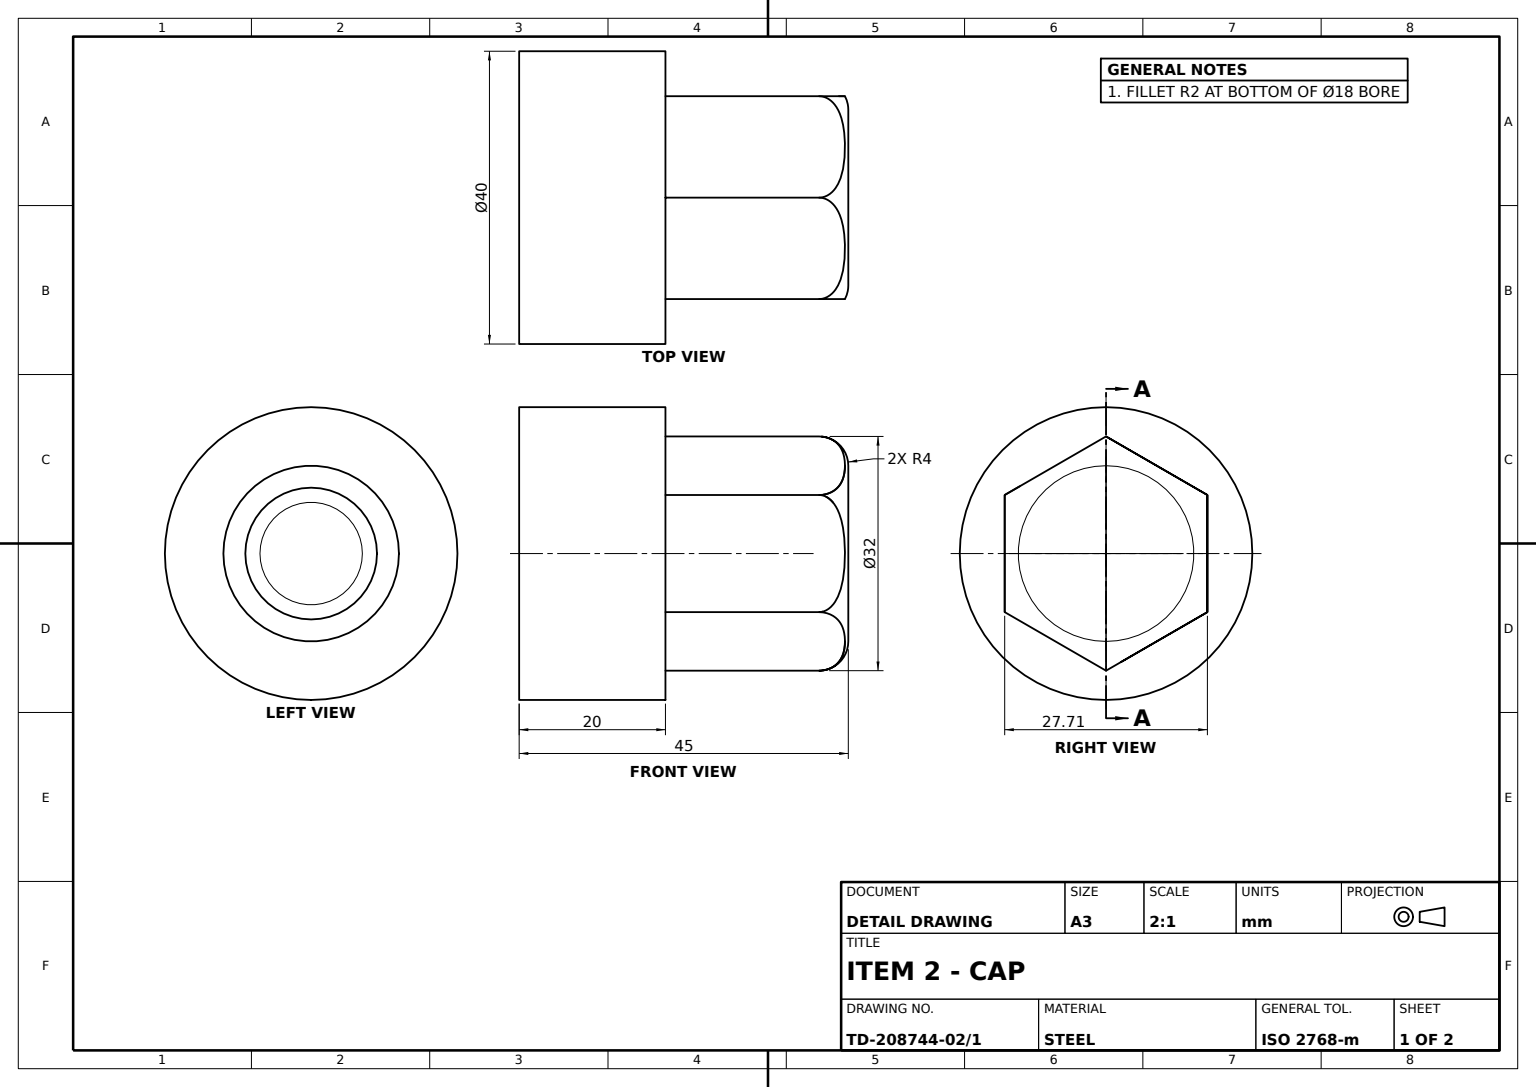
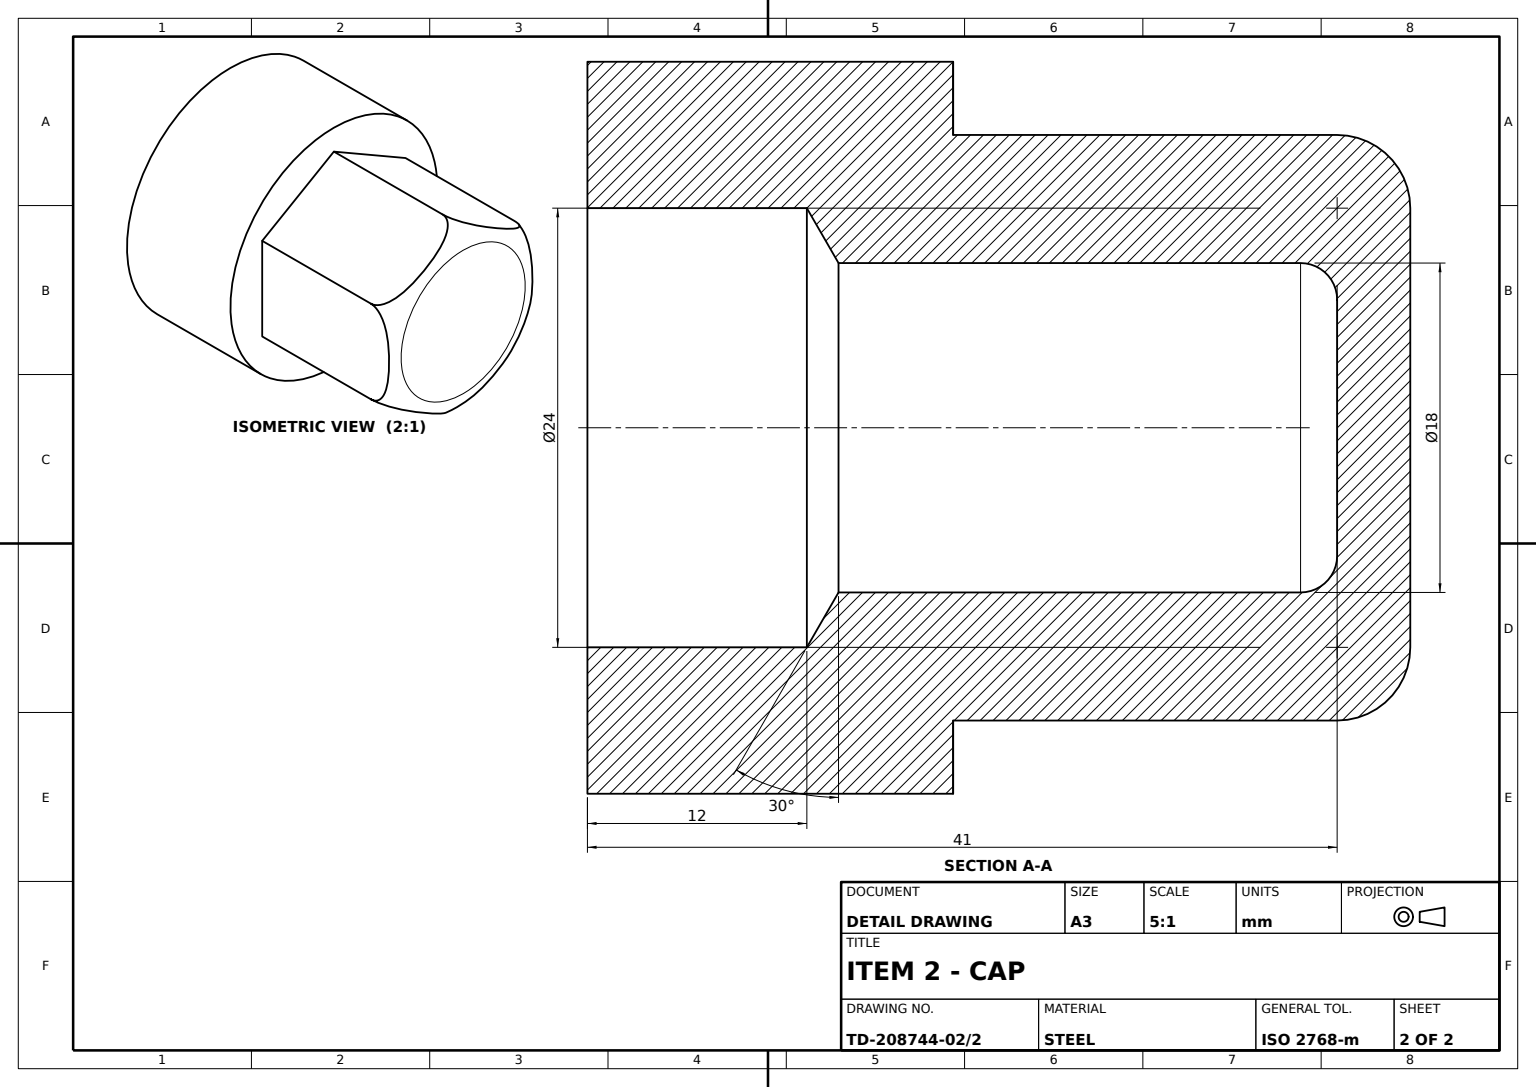
ISO-10303-21;
HEADER;
FILE_DESCRIPTION((''),'2;1');
FILE_NAME('','',(''),(''),'','','');
FILE_SCHEMA(('AUTOMOTIVE_DESIGN'));
ENDSEC;
DATA;
#1=APPLICATION_CONTEXT('');
#2=PRODUCT_CONTEXT('',#1,'mechanical');
#3=PRODUCT('','','',(#2));
#4=PRODUCT_DEFINITION_FORMATION('','',#3);
#5=PRODUCT_DEFINITION_CONTEXT('',#1,'design');
#6=PRODUCT_DEFINITION('','',#4,#5);
#7=PRODUCT_DEFINITION_SHAPE('','',#6);
#8=(LENGTH_UNIT()NAMED_UNIT(*)SI_UNIT(.MILLI.,.METRE.));
#9=(NAMED_UNIT(*)PLANE_ANGLE_UNIT()SI_UNIT($,.RADIAN.));
#10=(NAMED_UNIT(*)SI_UNIT($,.STERADIAN.)SOLID_ANGLE_UNIT());
#11=UNCERTAINTY_MEASURE_WITH_UNIT(LENGTH_MEASURE(1.E-05),#8,'distance_accuracy_value','');
#12=(GEOMETRIC_REPRESENTATION_CONTEXT(3)GLOBAL_UNCERTAINTY_ASSIGNED_CONTEXT((#11))GLOBAL_UNIT_ASSIGNED_CONTEXT((#8,#9,#10))REPRESENTATION_CONTEXT('',''));
#13=CARTESIAN_POINT('',(0.,0.,12.));
#14=VERTEX_POINT('',#13);
#15=CARTESIAN_POINT('',(0.,0.,-12.));
#16=VERTEX_POINT('',#15);
#17=CARTESIAN_POINT('',(0.,0.,0.));
#18=DIRECTION('',(0.,-1.,0.));
#19=DIRECTION('',(0.,0.,-1.));
#20=AXIS2_PLACEMENT_3D('',#17,#18,#19);
#21=CIRCLE('',#20,12.);
#22=EDGE_CURVE('',#14,#16,#21,.T.);
#23=ORIENTED_EDGE('',*,*,#22,.F.);
#24=EDGE_CURVE('',#16,#14,#21,.T.);
#25=ORIENTED_EDGE('',*,*,#24,.F.);
#26=EDGE_LOOP('',(#23,#25));
#27=FACE_BOUND('',#26,.T.);
#28=CARTESIAN_POINT('',(-20.,0.,0.));
#29=VERTEX_POINT('',#28);
#30=CARTESIAN_POINT('',(20.,0.,0.));
#31=VERTEX_POINT('',#30);
#32=DIRECTION('',(1.,0.,0.));
#33=AXIS2_PLACEMENT_3D('',#17,#18,#32);
#34=CIRCLE('',#33,20.);
#35=EDGE_CURVE('',#29,#31,#34,.T.);
#36=ORIENTED_EDGE('',*,*,#35,.T.);
#37=EDGE_CURVE('',#31,#29,#34,.T.);
#38=ORIENTED_EDGE('',*,*,#37,.T.);
#39=EDGE_LOOP('',(#36,#38));
#40=FACE_OUTER_BOUND('',#39,.T.);
#41=PLANE('',#33);
#42=ADVANCED_FACE('',(#27,#40),#41,.T.);
#43=CARTESIAN_POINT('',(0.,39.,-9.));
#44=VERTEX_POINT('',#43);
#45=CARTESIAN_POINT('',(0.,13.732051,-9.));
#46=VERTEX_POINT('',#45);
#47=CARTESIAN_POINT('',(0.,0.,-9.));
#48=VECTOR('',#18,1000.);
#49=LINE('',#47,#48);
#50=EDGE_CURVE('',#44,#46,#49,.T.);
#51=ORIENTED_EDGE('',*,*,#50,.T.);
#52=CARTESIAN_POINT('',(0.,13.732051,9.));
#53=VERTEX_POINT('',#52);
#54=CARTESIAN_POINT('',(0.,13.732051,0.));
#55=AXIS2_PLACEMENT_3D('',#54,#18,#19);
#56=CIRCLE('',#55,9.);
#57=EDGE_CURVE('',#46,#53,#56,.T.);
#58=ORIENTED_EDGE('',*,*,#57,.T.);
#59=CARTESIAN_POINT('',(0.,39.,9.));
#60=VERTEX_POINT('',#59);
#61=CARTESIAN_POINT('',(0.,0.,9.));
#62=LINE('',#61,#48);
#63=EDGE_CURVE('',#60,#53,#62,.T.);
#64=ORIENTED_EDGE('',*,*,#63,.F.);
#65=CARTESIAN_POINT('',(0.,39.,0.));
#66=AXIS2_PLACEMENT_3D('',#65,#18,#19);
#67=CIRCLE('',#66,9.);
#68=EDGE_CURVE('',#44,#60,#67,.T.);
#69=ORIENTED_EDGE('',*,*,#68,.F.);
#70=EDGE_LOOP('',(#51,#58,#64,#69));
#71=FACE_OUTER_BOUND('',#70,.T.);
#72=CYLINDRICAL_SURFACE('',#20,9.);
#73=ADVANCED_FACE('',(#71),#72,.F.);
#74=CARTESIAN_POINT('',(-12.,45.,0.));
#75=VERTEX_POINT('',#74);
#76=CARTESIAN_POINT('',(12.,45.,0.));
#77=VERTEX_POINT('',#76);
#78=CARTESIAN_POINT('',(0.,45.,0.));
#79=AXIS2_PLACEMENT_3D('',#78,#18,#32);
#80=CIRCLE('',#79,12.);
#81=EDGE_CURVE('',#75,#77,#80,.T.);
#82=ORIENTED_EDGE('',*,*,#81,.F.);
#83=EDGE_CURVE('',#77,#75,#80,.T.);
#84=ORIENTED_EDGE('',*,*,#83,.F.);
#85=EDGE_LOOP('',(#82,#84));
#86=FACE_OUTER_BOUND('',#85,.T.);
#87=DIRECTION('',(0.,1.,0.));
#88=DIRECTION('',(-1.,0.,0.));
#89=AXIS2_PLACEMENT_3D('',#76,#87,#88);
#90=PLANE('',#89);
#91=ADVANCED_FACE('',(#86),#90,.T.);
#92=CARTESIAN_POINT('',(-16.,20.,0.));
#93=VERTEX_POINT('',#92);
#94=CARTESIAN_POINT('',(-16.,41.,0.));
#95=VERTEX_POINT('',#94);
#96=VECTOR('',#87,1000.);
#97=LINE('',#92,#96);
#98=EDGE_CURVE('',#93,#95,#97,.T.);
#99=ORIENTED_EDGE('',*,*,#98,.T.);
#100=CARTESIAN_POINT('',(-8.,41.,-13.856406));
#101=VERTEX_POINT('',#100);
#102=CARTESIAN_POINT('',(-8.,41.202571,-13.856406));
#103=CARTESIAN_POINT('',(-8.015221,41.399792,-13.830042));
#104=CARTESIAN_POINT('',(-8.073295,41.784524,-13.729455));
#105=CARTESIAN_POINT('',(-8.115929,41.968487,-13.655611));
#106=CARTESIAN_POINT('',(-8.220838,42.310219,-13.473903));
#107=CARTESIAN_POINT('',(-8.283694,42.469836,-13.365034));
#108=CARTESIAN_POINT('',(-8.420692,42.759188,-13.127746));
#109=CARTESIAN_POINT('',(-8.495463,42.890957,-12.99824));
#110=CARTESIAN_POINT('',(-8.655022,43.133875,-12.721875));
#111=CARTESIAN_POINT('',(-8.739235,43.243922,-12.576014));
#112=CARTESIAN_POINT('',(-8.911565,43.442551,-12.27753));
#113=CARTESIAN_POINT('',(-9.000187,43.531843,-12.124032));
#114=CARTESIAN_POINT('',(-9.271939,43.775712,-11.653343));
#115=CARTESIAN_POINT('',(-9.462204,43.907128,-11.323795));
#116=CARTESIAN_POINT('',(-10.03618,44.22838,-10.329639));
#117=CARTESIAN_POINT('',(-10.425125,44.351502,-9.655968));
#118=CARTESIAN_POINT('',(-11.209098,44.509721,-8.298085));
#119=CARTESIAN_POINT('',(-11.605285,44.54321,-7.611869));
#120=CARTESIAN_POINT('',(-12.397477,44.543045,-6.239752));
#121=CARTESIAN_POINT('',(-12.791778,44.509605,-5.556804));
#122=CARTESIAN_POINT('',(-13.575458,44.351324,-4.199431));
#123=CARTESIAN_POINT('',(-13.964933,44.228271,-3.524839));
#124=CARTESIAN_POINT('',(-14.541664,43.904703,-2.525912));
#125=CARTESIAN_POINT('',(-14.730594,43.773933,-2.198675));
#126=CARTESIAN_POINT('',(-15.094705,43.446183,-1.568016));
#127=CARTESIAN_POINT('',(-15.26945,43.24963,-1.265349));
#128=CARTESIAN_POINT('',(-15.506279,42.887912,-0.85515));
#129=CARTESIAN_POINT('',(-15.581866,42.754452,-0.72423));
#130=CARTESIAN_POINT('',(-15.719001,42.463451,-0.486704));
#131=CARTESIAN_POINT('',(-15.780427,42.306728,-0.380312));
#132=CARTESIAN_POINT('',(-15.885052,41.964647,-0.199096));
#133=CARTESIAN_POINT('',(-15.927104,41.781816,-0.126259));
#134=CARTESIAN_POINT('',(-15.984323,41.402875,-0.027154));
#135=CARTESIAN_POINT('',(-16.,41.202181,0.));
#136=B_SPLINE_CURVE_WITH_KNOTS('',3,(#100,#102,#103,#104,#105,#106,#107,#108,#109,#110,#111,#112,#113,#114,#115,#116,#117,#118,#119,#120,#121,#122,#123,#124,#125,#126,#127,#128,#129,#130,#131,#132,#133,#134,#135,#94),.UNSPECIFIED.,.F.,.F.,(4,2,2,2,2,2,2,2,2,2,2,2,2,2,2,2,2,4),(0.000000197,0.000598739,0.00119728,0.001795822,0.002394364,0.002992905,0.003591447,0.00478853,0.007182697,0.009576864,0.01197103,0.014365197,0.01556228,0.016759364,0.017357905,0.017956447,0.018554989,0.01915353),.UNSPECIFIED.);
#137=EDGE_CURVE('',#101,#95,#136,.T.);
#138=ORIENTED_EDGE('',*,*,#137,.F.);
#139=CARTESIAN_POINT('',(-8.,20.,-13.856406));
#140=VERTEX_POINT('',#139);
#141=LINE('',#139,#96);
#142=EDGE_CURVE('',#140,#101,#141,.T.);
#143=ORIENTED_EDGE('',*,*,#142,.F.);
#144=DIRECTION('',(-0.5,0.,0.866025404));
#145=VECTOR('',#144,1000.);
#146=LINE('',#139,#145);
#147=EDGE_CURVE('',#140,#93,#146,.T.);
#148=ORIENTED_EDGE('',*,*,#147,.T.);
#149=EDGE_LOOP('',(#99,#138,#143,#148));
#150=FACE_OUTER_BOUND('',#149,.T.);
#151=DIRECTION('',(-0.866025404,0.,-0.5));
#152=AXIS2_PLACEMENT_3D('',#139,#151,#144);
#153=PLANE('',#152);
#154=ADVANCED_FACE('',(#150),#153,.T.);
#155=CARTESIAN_POINT('',(0.,12.,12.));
#156=VERTEX_POINT('',#155);
#157=LINE('',#13,#48);
#158=EDGE_CURVE('',#156,#14,#157,.T.);
#159=ORIENTED_EDGE('',*,*,#158,.T.);
#160=ORIENTED_EDGE('',*,*,#22,.T.);
#161=CARTESIAN_POINT('',(0.,12.,-12.));
#162=VERTEX_POINT('',#161);
#163=LINE('',#15,#48);
#164=EDGE_CURVE('',#162,#16,#163,.T.);
#165=ORIENTED_EDGE('',*,*,#164,.F.);
#166=CARTESIAN_POINT('',(0.,12.,0.));
#167=AXIS2_PLACEMENT_3D('',#166,#18,#19);
#168=CIRCLE('',#167,12.);
#169=EDGE_CURVE('',#156,#162,#168,.T.);
#170=ORIENTED_EDGE('',*,*,#169,.F.);
#171=EDGE_LOOP('',(#159,#160,#165,#170));
#172=FACE_OUTER_BOUND('',#171,.T.);
#173=CYLINDRICAL_SURFACE('',#20,12.);
#174=ADVANCED_FACE('',(#172),#173,.F.);
#175=CARTESIAN_POINT('',(-12.,41.,0.));
#176=DIRECTION('',(0.,0.,1.));
#177=AXIS2_PLACEMENT_3D('',#175,#176,#32);
#178=CIRCLE('',#177,4.);
#179=EDGE_CURVE('',#75,#95,#178,.T.);
#180=ORIENTED_EDGE('',*,*,#179,.F.);
#181=ORIENTED_EDGE('',*,*,#81,.T.);
#182=CARTESIAN_POINT('',(16.,41.,0.));
#183=VERTEX_POINT('',#182);
#184=CARTESIAN_POINT('',(12.,41.,0.));
#185=AXIS2_PLACEMENT_3D('',#184,#19,#88);
#186=CIRCLE('',#185,4.);
#187=EDGE_CURVE('',#77,#183,#186,.T.);
#188=ORIENTED_EDGE('',*,*,#187,.T.);
#189=CARTESIAN_POINT('',(8.,41.,-13.856406));
#190=VERTEX_POINT('',#189);
#191=CARTESIAN_POINT('',(16.,41.202571,0.));
#192=CARTESIAN_POINT('',(15.984779,41.399792,-0.026364));
#193=CARTESIAN_POINT('',(15.926705,41.784524,-0.126951));
#194=CARTESIAN_POINT('',(15.884071,41.968487,-0.200795));
#195=CARTESIAN_POINT('',(15.779162,42.310219,-0.382503));
#196=CARTESIAN_POINT('',(15.716306,42.469836,-0.491372));
#197=CARTESIAN_POINT('',(15.579308,42.759188,-0.728661));
#198=CARTESIAN_POINT('',(15.504537,42.890957,-0.858166));
#199=CARTESIAN_POINT('',(15.344978,43.133875,-1.134531));
#200=CARTESIAN_POINT('',(15.260765,43.243922,-1.280392));
#201=CARTESIAN_POINT('',(15.088435,43.442551,-1.578876));
#202=CARTESIAN_POINT('',(14.999813,43.531843,-1.732375));
#203=CARTESIAN_POINT('',(14.728061,43.775712,-2.203064));
#204=CARTESIAN_POINT('',(14.537796,43.907128,-2.532611));
#205=CARTESIAN_POINT('',(13.96382,44.22838,-3.526767));
#206=CARTESIAN_POINT('',(13.574875,44.351502,-4.200439));
#207=CARTESIAN_POINT('',(12.790902,44.509721,-5.558321));
#208=CARTESIAN_POINT('',(12.394715,44.54321,-6.244537));
#209=CARTESIAN_POINT('',(11.602523,44.543045,-7.616654));
#210=CARTESIAN_POINT('',(11.208222,44.509605,-8.299602));
#211=CARTESIAN_POINT('',(10.424542,44.351324,-9.656976));
#212=CARTESIAN_POINT('',(10.035067,44.228271,-10.331568));
#213=CARTESIAN_POINT('',(9.458336,43.904703,-11.330495));
#214=CARTESIAN_POINT('',(9.269406,43.773933,-11.657731));
#215=CARTESIAN_POINT('',(8.905295,43.446183,-12.28839));
#216=CARTESIAN_POINT('',(8.73055,43.24963,-12.591057));
#217=CARTESIAN_POINT('',(8.493721,42.887912,-13.001257));
#218=CARTESIAN_POINT('',(8.418134,42.754452,-13.132177));
#219=CARTESIAN_POINT('',(8.280999,42.463451,-13.369702));
#220=CARTESIAN_POINT('',(8.219573,42.306728,-13.476094));
#221=CARTESIAN_POINT('',(8.114948,41.964647,-13.657311));
#222=CARTESIAN_POINT('',(8.072896,41.781816,-13.730147));
#223=CARTESIAN_POINT('',(8.015677,41.402875,-13.829253));
#224=CARTESIAN_POINT('',(8.,41.202181,-13.856406));
#225=B_SPLINE_CURVE_WITH_KNOTS('',3,(#182,#191,#192,#193,#194,#195,#196,#197,#198,#199,#200,#201,#202,#203,#204,#205,#206,#207,#208,#209,#210,#211,#212,#213,#214,#215,#216,#217,#218,#219,#220,#221,#222,#223,#224,#189),.UNSPECIFIED.,.F.,.F.,(4,2,2,2,2,2,2,2,2,2,2,2,2,2,2,2,2,4),(0.000000197,0.000598739,0.00119728,0.001795822,0.002394364,0.002992905,0.003591447,0.00478853,0.007182697,0.009576864,0.01197103,0.014365197,0.01556228,0.016759364,0.017357905,0.017956447,0.018554989,0.01915353),.UNSPECIFIED.);
#226=EDGE_CURVE('',#183,#190,#225,.T.);
#227=ORIENTED_EDGE('',*,*,#226,.T.);
#228=CARTESIAN_POINT('',(8.,41.198735,-13.856406));
#229=CARTESIAN_POINT('',(7.9694,41.400114,-13.856406));
#230=CARTESIAN_POINT('',(7.853924,41.783017,-13.856406));
#231=CARTESIAN_POINT('',(7.769066,41.966653,-13.856406));
#232=CARTESIAN_POINT('',(7.559712,42.308282,-13.856406));
#233=CARTESIAN_POINT('',(7.436968,42.464642,-13.856406));
#234=CARTESIAN_POINT('',(7.1633,42.754815,-13.856406));
#235=CARTESIAN_POINT('',(7.011682,42.888658,-13.856406));
#236=CARTESIAN_POINT('',(6.537566,43.250493,-13.856406));
#237=CARTESIAN_POINT('',(6.190168,43.445805,-13.856406));
#238=CARTESIAN_POINT('',(5.461456,43.77385,-13.856406));
#239=CARTESIAN_POINT('',(5.08742,43.90319,-13.856406));
#240=CARTESIAN_POINT('',(3.946634,44.224285,-13.856406));
#241=CARTESIAN_POINT('',(3.15796,44.350566,-13.856406));
#242=CARTESIAN_POINT('',(1.578733,44.510138,-13.856406));
#243=CARTESIAN_POINT('',(0.78461,44.5434,-13.856406));
#244=CARTESIAN_POINT('',(-0.802861,44.542852,-13.856406));
#245=CARTESIAN_POINT('',(-1.59343,44.509118,-13.856406));
#246=CARTESIAN_POINT('',(-2.772732,44.389254,-13.856406));
#247=CARTESIAN_POINT('',(-3.164704,44.33737,-13.856406));
#248=CARTESIAN_POINT('',(-3.945518,44.200532,-13.856406));
#249=CARTESIAN_POINT('',(-4.335639,44.115248,-13.856406));
#250=CARTESIAN_POINT('',(-5.099799,43.899237,-13.856406));
#251=CARTESIAN_POINT('',(-5.476244,43.768117,-13.856406));
#252=CARTESIAN_POINT('',(-6.201131,43.439912,-13.856406));
#253=CARTESIAN_POINT('',(-6.544803,43.245806,-13.856406));
#254=CARTESIAN_POINT('',(-7.016468,42.884577,-13.856406));
#255=CARTESIAN_POINT('',(-7.167531,42.750827,-13.856406));
#256=CARTESIAN_POINT('',(-7.440539,42.460343,-13.856406));
#257=CARTESIAN_POINT('',(-7.563092,42.303669,-13.856406));
#258=CARTESIAN_POINT('',(-7.772114,41.960748,-13.856406));
#259=CARTESIAN_POINT('',(-7.855077,41.779661,-13.856406));
#260=CARTESIAN_POINT('',(-7.969095,41.400653,-13.856406));
#261=CARTESIAN_POINT('',(-8.,41.198468,-13.856406));
#262=B_SPLINE_CURVE_WITH_KNOTS('',3,(#189,#228,#229,#230,#231,#232,#233,#234,#235,#236,#237,#238,#239,#240,#241,#242,#243,#244,#245,#246,#247,#248,#249,#250,#251,#252,#253,#254,#255,#256,#257,#258,#259,#260,#261,#100),.UNSPECIFIED.,.F.,.F.,(4,2,2,2,2,2,2,2,2,2,2,2,2,2,2,2,2,4),(0.028497176,0.029089851,0.029682525,0.030275199,0.030867874,0.032053222,0.033238571,0.035609268,0.037979965,0.040350662,0.04153601,0.042721359,0.043906707,0.045092056,0.04568473,0.046277405,0.046870079,0.047462753),.UNSPECIFIED.);
#263=EDGE_CURVE('',#190,#101,#262,.T.);
#264=ORIENTED_EDGE('',*,*,#263,.T.);
#265=ORIENTED_EDGE('',*,*,#137,.T.);
#266=EDGE_LOOP('',(#180,#181,#188,#227,#264,#265));
#267=FACE_OUTER_BOUND('',#266,.T.);
#268=CARTESIAN_POINT('',(0.,41.,0.));
#269=AXIS2_PLACEMENT_3D('',#268,#18,#32);
#270=TOROIDAL_SURFACE('',#269,12.,4.);
#271=ADVANCED_FACE('',(#267),#270,.T.);
#272=CARTESIAN_POINT('',(0.,41.,7.));
#273=VERTEX_POINT('',#272);
#274=CARTESIAN_POINT('',(0.,39.,7.));
#275=AXIS2_PLACEMENT_3D('',#274,#32,#19);
#276=CIRCLE('',#275,2.);
#277=EDGE_CURVE('',#273,#60,#276,.T.);
#278=ORIENTED_EDGE('',*,*,#277,.T.);
#279=EDGE_CURVE('',#60,#44,#67,.T.);
#280=ORIENTED_EDGE('',*,*,#279,.T.);
#281=CARTESIAN_POINT('',(0.,41.,-7.));
#282=VERTEX_POINT('',#281);
#283=CARTESIAN_POINT('',(0.,39.,-7.));
#284=AXIS2_PLACEMENT_3D('',#283,#88,#176);
#285=CIRCLE('',#284,2.);
#286=EDGE_CURVE('',#282,#44,#285,.T.);
#287=ORIENTED_EDGE('',*,*,#286,.F.);
#288=AXIS2_PLACEMENT_3D('',#268,#18,#19);
#289=CIRCLE('',#288,7.);
#290=EDGE_CURVE('',#273,#282,#289,.T.);
#291=ORIENTED_EDGE('',*,*,#290,.F.);
#292=EDGE_LOOP('',(#278,#280,#287,#291));
#293=FACE_OUTER_BOUND('',#292,.T.);
#294=TOROIDAL_SURFACE('',#66,7.,2.);
#295=ADVANCED_FACE('',(#293),#294,.F.);
#296=CARTESIAN_POINT('',(8.,20.,-13.856406));
#297=VERTEX_POINT('',#296);
#298=VECTOR('',#88,1000.);
#299=LINE('',#296,#298);
#300=EDGE_CURVE('',#297,#140,#299,.T.);
#301=ORIENTED_EDGE('',*,*,#300,.T.);
#302=ORIENTED_EDGE('',*,*,#142,.T.);
#303=ORIENTED_EDGE('',*,*,#263,.F.);
#304=LINE('',#296,#96);
#305=EDGE_CURVE('',#297,#190,#304,.T.);
#306=ORIENTED_EDGE('',*,*,#305,.F.);
#307=EDGE_LOOP('',(#301,#302,#303,#306));
#308=FACE_OUTER_BOUND('',#307,.T.);
#309=AXIS2_PLACEMENT_3D('',#296,#19,#88);
#310=PLANE('',#309);
#311=ADVANCED_FACE('',(#308),#310,.T.);
#312=EDGE_CURVE('',#162,#156,#168,.T.);
#313=ORIENTED_EDGE('',*,*,#312,.T.);
#314=DIRECTION('',(0.,-0.5,0.866025404));
#315=VECTOR('',#314,1000.);
#316=LINE('',#155,#315);
#317=EDGE_CURVE('',#53,#156,#316,.T.);
#318=ORIENTED_EDGE('',*,*,#317,.F.);
#319=ORIENTED_EDGE('',*,*,#57,.F.);
#320=DIRECTION('',(0.,-0.5,-0.866025404));
#321=VECTOR('',#320,1000.);
#322=LINE('',#161,#321);
#323=EDGE_CURVE('',#46,#162,#322,.T.);
#324=ORIENTED_EDGE('',*,*,#323,.T.);
#325=EDGE_LOOP('',(#313,#318,#319,#324));
#326=FACE_OUTER_BOUND('',#325,.T.);
#327=CONICAL_SURFACE('',#167,12.,1.047197551);
#328=ADVANCED_FACE('',(#326),#327,.F.);
#329=ORIENTED_EDGE('',*,*,#169,.T.);
#330=ORIENTED_EDGE('',*,*,#323,.F.);
#331=EDGE_CURVE('',#53,#46,#56,.T.);
#332=ORIENTED_EDGE('',*,*,#331,.F.);
#333=ORIENTED_EDGE('',*,*,#317,.T.);
#334=EDGE_LOOP('',(#329,#330,#332,#333));
#335=FACE_OUTER_BOUND('',#334,.T.);
#336=ADVANCED_FACE('',(#335),#327,.F.);
#337=CARTESIAN_POINT('',(16.,20.,0.));
#338=VERTEX_POINT('',#337);
#339=LINE('',#337,#96);
#340=EDGE_CURVE('',#338,#183,#339,.T.);
#341=ORIENTED_EDGE('',*,*,#340,.F.);
#342=DIRECTION('',(-0.5,0.,-0.866025404));
#343=VECTOR('',#342,1000.);
#344=LINE('',#337,#343);
#345=EDGE_CURVE('',#338,#297,#344,.T.);
#346=ORIENTED_EDGE('',*,*,#345,.T.);
#347=ORIENTED_EDGE('',*,*,#305,.T.);
#348=ORIENTED_EDGE('',*,*,#226,.F.);
#349=EDGE_LOOP('',(#341,#346,#347,#348));
#350=FACE_OUTER_BOUND('',#349,.T.);
#351=DIRECTION('',(0.866025404,0.,-0.5));
#352=AXIS2_PLACEMENT_3D('',#337,#351,#342);
#353=PLANE('',#352);
#354=ADVANCED_FACE('',(#350),#353,.T.);
#355=CARTESIAN_POINT('',(-20.,20.,0.));
#356=VERTEX_POINT('',#355);
#357=CARTESIAN_POINT('',(20.,20.,0.));
#358=VERTEX_POINT('',#357);
#359=CARTESIAN_POINT('',(0.,20.,0.));
#360=AXIS2_PLACEMENT_3D('',#359,#18,#32);
#361=CIRCLE('',#360,20.);
#362=EDGE_CURVE('',#356,#358,#361,.T.);
#363=ORIENTED_EDGE('',*,*,#362,.T.);
#364=LINE('',#30,#48);
#365=EDGE_CURVE('',#358,#31,#364,.T.);
#366=ORIENTED_EDGE('',*,*,#365,.T.);
#367=ORIENTED_EDGE('',*,*,#35,.F.);
#368=LINE('',#28,#48);
#369=EDGE_CURVE('',#356,#29,#368,.T.);
#370=ORIENTED_EDGE('',*,*,#369,.F.);
#371=EDGE_LOOP('',(#363,#366,#367,#370));
#372=FACE_OUTER_BOUND('',#371,.T.);
#373=CYLINDRICAL_SURFACE('',#33,20.);
#374=ADVANCED_FACE('',(#372),#373,.T.);
#375=ORIENTED_EDGE('',*,*,#286,.T.);
#376=ORIENTED_EDGE('',*,*,#68,.T.);
#377=ORIENTED_EDGE('',*,*,#277,.F.);
#378=EDGE_CURVE('',#282,#273,#289,.T.);
#379=ORIENTED_EDGE('',*,*,#378,.F.);
#380=EDGE_LOOP('',(#375,#376,#377,#379));
#381=FACE_OUTER_BOUND('',#380,.T.);
#382=ADVANCED_FACE('',(#381),#294,.F.);
#383=CARTESIAN_POINT('',(-8.,41.,13.856406));
#384=VERTEX_POINT('',#383);
#385=CARTESIAN_POINT('',(-16.,41.202571,0.));
#386=CARTESIAN_POINT('',(-15.984779,41.399792,0.026364));
#387=CARTESIAN_POINT('',(-15.926705,41.784524,0.126951));
#388=CARTESIAN_POINT('',(-15.884071,41.968487,0.200795));
#389=CARTESIAN_POINT('',(-15.779162,42.310219,0.382503));
#390=CARTESIAN_POINT('',(-15.716306,42.469836,0.491372));
#391=CARTESIAN_POINT('',(-15.579308,42.759188,0.728661));
#392=CARTESIAN_POINT('',(-15.504537,42.890957,0.858166));
#393=CARTESIAN_POINT('',(-15.344978,43.133875,1.134531));
#394=CARTESIAN_POINT('',(-15.260765,43.243922,1.280392));
#395=CARTESIAN_POINT('',(-15.088435,43.442551,1.578876));
#396=CARTESIAN_POINT('',(-14.999813,43.531843,1.732375));
#397=CARTESIAN_POINT('',(-14.728061,43.775712,2.203064));
#398=CARTESIAN_POINT('',(-14.537796,43.907128,2.532611));
#399=CARTESIAN_POINT('',(-13.96382,44.22838,3.526767));
#400=CARTESIAN_POINT('',(-13.574875,44.351502,4.200439));
#401=CARTESIAN_POINT('',(-12.790902,44.509721,5.558321));
#402=CARTESIAN_POINT('',(-12.394715,44.54321,6.244537));
#403=CARTESIAN_POINT('',(-11.602523,44.543045,7.616654));
#404=CARTESIAN_POINT('',(-11.208222,44.509605,8.299602));
#405=CARTESIAN_POINT('',(-10.424542,44.351324,9.656976));
#406=CARTESIAN_POINT('',(-10.035067,44.228271,10.331568));
#407=CARTESIAN_POINT('',(-9.458336,43.904703,11.330495));
#408=CARTESIAN_POINT('',(-9.269406,43.773933,11.657731));
#409=CARTESIAN_POINT('',(-8.905295,43.446183,12.28839));
#410=CARTESIAN_POINT('',(-8.73055,43.24963,12.591057));
#411=CARTESIAN_POINT('',(-8.493721,42.887912,13.001257));
#412=CARTESIAN_POINT('',(-8.418134,42.754452,13.132177));
#413=CARTESIAN_POINT('',(-8.280999,42.463451,13.369702));
#414=CARTESIAN_POINT('',(-8.219573,42.306728,13.476094));
#415=CARTESIAN_POINT('',(-8.114948,41.964647,13.657311));
#416=CARTESIAN_POINT('',(-8.072896,41.781816,13.730147));
#417=CARTESIAN_POINT('',(-8.015677,41.402875,13.829253));
#418=CARTESIAN_POINT('',(-8.,41.202181,13.856406));
#419=B_SPLINE_CURVE_WITH_KNOTS('',3,(#94,#385,#386,#387,#388,#389,#390,#391,#392,#393,#394,#395,#396,#397,#398,#399,#400,#401,#402,#403,#404,#405,#406,#407,#408,#409,#410,#411,#412,#413,#414,#415,#416,#417,#418,#383),.UNSPECIFIED.,.F.,.F.,(4,2,2,2,2,2,2,2,2,2,2,2,2,2,2,2,2,4),(0.000000197,0.000598739,0.00119728,0.001795822,0.002394364,0.002992905,0.003591447,0.00478853,0.007182697,0.009576864,0.01197103,0.014365197,0.01556228,0.016759364,0.017357905,0.017956447,0.018554989,0.01915353),.UNSPECIFIED.);
#420=EDGE_CURVE('',#95,#384,#419,.T.);
#421=ORIENTED_EDGE('',*,*,#420,.T.);
#422=CARTESIAN_POINT('',(8.,41.,13.856406));
#423=VERTEX_POINT('',#422);
#424=CARTESIAN_POINT('',(-8.,41.198735,13.856406));
#425=CARTESIAN_POINT('',(-7.9694,41.400114,13.856406));
#426=CARTESIAN_POINT('',(-7.853924,41.783017,13.856406));
#427=CARTESIAN_POINT('',(-7.769066,41.966653,13.856406));
#428=CARTESIAN_POINT('',(-7.559712,42.308282,13.856406));
#429=CARTESIAN_POINT('',(-7.436968,42.464642,13.856406));
#430=CARTESIAN_POINT('',(-7.1633,42.754815,13.856406));
#431=CARTESIAN_POINT('',(-7.011682,42.888658,13.856406));
#432=CARTESIAN_POINT('',(-6.537566,43.250493,13.856406));
#433=CARTESIAN_POINT('',(-6.190168,43.445805,13.856406));
#434=CARTESIAN_POINT('',(-5.461456,43.77385,13.856406));
#435=CARTESIAN_POINT('',(-5.08742,43.90319,13.856406));
#436=CARTESIAN_POINT('',(-3.946634,44.224285,13.856406));
#437=CARTESIAN_POINT('',(-3.15796,44.350566,13.856406));
#438=CARTESIAN_POINT('',(-1.578733,44.510138,13.856406));
#439=CARTESIAN_POINT('',(-0.78461,44.5434,13.856406));
#440=CARTESIAN_POINT('',(0.802861,44.542852,13.856406));
#441=CARTESIAN_POINT('',(1.59343,44.509118,13.856406));
#442=CARTESIAN_POINT('',(2.772732,44.389254,13.856406));
#443=CARTESIAN_POINT('',(3.164704,44.33737,13.856406));
#444=CARTESIAN_POINT('',(3.945518,44.200532,13.856406));
#445=CARTESIAN_POINT('',(4.335639,44.115248,13.856406));
#446=CARTESIAN_POINT('',(5.099799,43.899237,13.856406));
#447=CARTESIAN_POINT('',(5.476244,43.768117,13.856406));
#448=CARTESIAN_POINT('',(6.201131,43.439912,13.856406));
#449=CARTESIAN_POINT('',(6.544803,43.245806,13.856406));
#450=CARTESIAN_POINT('',(7.016468,42.884577,13.856406));
#451=CARTESIAN_POINT('',(7.167531,42.750827,13.856406));
#452=CARTESIAN_POINT('',(7.440539,42.460343,13.856406));
#453=CARTESIAN_POINT('',(7.563092,42.303669,13.856406));
#454=CARTESIAN_POINT('',(7.772114,41.960748,13.856406));
#455=CARTESIAN_POINT('',(7.855077,41.779661,13.856406));
#456=CARTESIAN_POINT('',(7.969095,41.400653,13.856406));
#457=CARTESIAN_POINT('',(8.,41.198468,13.856406));
#458=B_SPLINE_CURVE_WITH_KNOTS('',3,(#383,#424,#425,#426,#427,#428,#429,#430,#431,#432,#433,#434,#435,#436,#437,#438,#439,#440,#441,#442,#443,#444,#445,#446,#447,#448,#449,#450,#451,#452,#453,#454,#455,#456,#457,#422),.UNSPECIFIED.,.F.,.F.,(4,2,2,2,2,2,2,2,2,2,2,2,2,2,2,2,2,4),(0.028497176,0.029089851,0.029682525,0.030275199,0.030867874,0.032053222,0.033238571,0.035609268,0.037979965,0.040350662,0.04153601,0.042721359,0.043906707,0.045092056,0.04568473,0.046277405,0.046870079,0.047462753),.UNSPECIFIED.);
#459=EDGE_CURVE('',#384,#423,#458,.T.);
#460=ORIENTED_EDGE('',*,*,#459,.T.);
#461=CARTESIAN_POINT('',(8.,41.202571,13.856406));
#462=CARTESIAN_POINT('',(8.015221,41.399792,13.830042));
#463=CARTESIAN_POINT('',(8.073295,41.784524,13.729455));
#464=CARTESIAN_POINT('',(8.115929,41.968487,13.655611));
#465=CARTESIAN_POINT('',(8.220838,42.310219,13.473903));
#466=CARTESIAN_POINT('',(8.283694,42.469836,13.365034));
#467=CARTESIAN_POINT('',(8.420692,42.759188,13.127746));
#468=CARTESIAN_POINT('',(8.495463,42.890957,12.99824));
#469=CARTESIAN_POINT('',(8.655022,43.133875,12.721875));
#470=CARTESIAN_POINT('',(8.739235,43.243922,12.576014));
#471=CARTESIAN_POINT('',(8.911565,43.442551,12.27753));
#472=CARTESIAN_POINT('',(9.000187,43.531843,12.124032));
#473=CARTESIAN_POINT('',(9.271939,43.775712,11.653343));
#474=CARTESIAN_POINT('',(9.462204,43.907128,11.323795));
#475=CARTESIAN_POINT('',(10.03618,44.22838,10.329639));
#476=CARTESIAN_POINT('',(10.425125,44.351502,9.655968));
#477=CARTESIAN_POINT('',(11.209098,44.509721,8.298085));
#478=CARTESIAN_POINT('',(11.605285,44.54321,7.611869));
#479=CARTESIAN_POINT('',(12.397477,44.543045,6.239752));
#480=CARTESIAN_POINT('',(12.791778,44.509605,5.556804));
#481=CARTESIAN_POINT('',(13.575458,44.351324,4.199431));
#482=CARTESIAN_POINT('',(13.964933,44.228271,3.524839));
#483=CARTESIAN_POINT('',(14.541664,43.904703,2.525912));
#484=CARTESIAN_POINT('',(14.730594,43.773933,2.198675));
#485=CARTESIAN_POINT('',(15.094705,43.446183,1.568016));
#486=CARTESIAN_POINT('',(15.26945,43.24963,1.265349));
#487=CARTESIAN_POINT('',(15.506279,42.887912,0.85515));
#488=CARTESIAN_POINT('',(15.581866,42.754452,0.72423));
#489=CARTESIAN_POINT('',(15.719001,42.463451,0.486704));
#490=CARTESIAN_POINT('',(15.780427,42.306728,0.380312));
#491=CARTESIAN_POINT('',(15.885052,41.964647,0.199096));
#492=CARTESIAN_POINT('',(15.927104,41.781816,0.126259));
#493=CARTESIAN_POINT('',(15.984323,41.402875,0.027154));
#494=CARTESIAN_POINT('',(16.,41.202181,0.));
#495=B_SPLINE_CURVE_WITH_KNOTS('',3,(#422,#461,#462,#463,#464,#465,#466,#467,#468,#469,#470,#471,#472,#473,#474,#475,#476,#477,#478,#479,#480,#481,#482,#483,#484,#485,#486,#487,#488,#489,#490,#491,#492,#493,#494,#182),.UNSPECIFIED.,.F.,.F.,(4,2,2,2,2,2,2,2,2,2,2,2,2,2,2,2,2,4),(0.000000197,0.000598739,0.00119728,0.001795822,0.002394364,0.002992905,0.003591447,0.00478853,0.007182697,0.009576864,0.01197103,0.014365197,0.01556228,0.016759364,0.017357905,0.017956447,0.018554989,0.01915353),.UNSPECIFIED.);
#496=EDGE_CURVE('',#423,#183,#495,.T.);
#497=ORIENTED_EDGE('',*,*,#496,.T.);
#498=ORIENTED_EDGE('',*,*,#187,.F.);
#499=ORIENTED_EDGE('',*,*,#83,.T.);
#500=ORIENTED_EDGE('',*,*,#179,.T.);
#501=EDGE_LOOP('',(#421,#460,#497,#498,#499,#500));
#502=FACE_OUTER_BOUND('',#501,.T.);
#503=ADVANCED_FACE('',(#502),#270,.T.);
#504=ORIENTED_EDGE('',*,*,#420,.F.);
#505=ORIENTED_EDGE('',*,*,#98,.F.);
#506=CARTESIAN_POINT('',(-8.,20.,13.856406));
#507=VERTEX_POINT('',#506);
#508=DIRECTION('',(0.5,0.,0.866025404));
#509=VECTOR('',#508,1000.);
#510=LINE('',#92,#509);
#511=EDGE_CURVE('',#93,#507,#510,.T.);
#512=ORIENTED_EDGE('',*,*,#511,.T.);
#513=LINE('',#506,#96);
#514=EDGE_CURVE('',#507,#384,#513,.T.);
#515=ORIENTED_EDGE('',*,*,#514,.T.);
#516=EDGE_LOOP('',(#504,#505,#512,#515));
#517=FACE_OUTER_BOUND('',#516,.T.);
#518=DIRECTION('',(-0.866025404,0.,0.5));
#519=AXIS2_PLACEMENT_3D('',#92,#518,#508);
#520=PLANE('',#519);
#521=ADVANCED_FACE('',(#517),#520,.T.);
#522=ORIENTED_EDGE('',*,*,#378,.T.);
#523=ORIENTED_EDGE('',*,*,#290,.T.);
#524=EDGE_LOOP('',(#522,#523));
#525=FACE_OUTER_BOUND('',#524,.T.);
#526=CARTESIAN_POINT('',(7.,41.,0.));
#527=AXIS2_PLACEMENT_3D('',#526,#87,#176);
#528=PLANE('',#527);
#529=ADVANCED_FACE('',(#525),#528,.F.);
#530=ORIENTED_EDGE('',*,*,#164,.T.);
#531=ORIENTED_EDGE('',*,*,#24,.T.);
#532=ORIENTED_EDGE('',*,*,#158,.F.);
#533=ORIENTED_EDGE('',*,*,#312,.F.);
#534=EDGE_LOOP('',(#530,#531,#532,#533));
#535=FACE_OUTER_BOUND('',#534,.T.);
#536=ADVANCED_FACE('',(#535),#173,.F.);
#537=CARTESIAN_POINT('',(8.,20.,13.856406));
#538=VERTEX_POINT('',#537);
#539=DIRECTION('',(0.5,0.,-0.866025404));
#540=VECTOR('',#539,1000.);
#541=LINE('',#537,#540);
#542=EDGE_CURVE('',#538,#338,#541,.T.);
#543=ORIENTED_EDGE('',*,*,#542,.F.);
#544=VECTOR('',#32,1000.);
#545=LINE('',#506,#544);
#546=EDGE_CURVE('',#507,#538,#545,.T.);
#547=ORIENTED_EDGE('',*,*,#546,.F.);
#548=ORIENTED_EDGE('',*,*,#511,.F.);
#549=ORIENTED_EDGE('',*,*,#147,.F.);
#550=ORIENTED_EDGE('',*,*,#300,.F.);
#551=ORIENTED_EDGE('',*,*,#345,.F.);
#552=EDGE_LOOP('',(#543,#547,#548,#549,#550,#551));
#553=FACE_BOUND('',#552,.T.);
#554=ORIENTED_EDGE('',*,*,#362,.F.);
#555=EDGE_CURVE('',#358,#356,#361,.T.);
#556=ORIENTED_EDGE('',*,*,#555,.F.);
#557=EDGE_LOOP('',(#554,#556));
#558=FACE_OUTER_BOUND('',#557,.T.);
#559=AXIS2_PLACEMENT_3D('',#357,#87,#88);
#560=PLANE('',#559);
#561=ADVANCED_FACE('',(#553,#558),#560,.T.);
#562=ORIENTED_EDGE('',*,*,#37,.F.);
#563=ORIENTED_EDGE('',*,*,#365,.F.);
#564=ORIENTED_EDGE('',*,*,#555,.T.);
#565=ORIENTED_EDGE('',*,*,#369,.T.);
#566=EDGE_LOOP('',(#562,#563,#564,#565));
#567=FACE_OUTER_BOUND('',#566,.T.);
#568=ADVANCED_FACE('',(#567),#373,.T.);
#569=ORIENTED_EDGE('',*,*,#542,.T.);
#570=ORIENTED_EDGE('',*,*,#340,.T.);
#571=ORIENTED_EDGE('',*,*,#496,.F.);
#572=LINE('',#537,#96);
#573=EDGE_CURVE('',#538,#423,#572,.T.);
#574=ORIENTED_EDGE('',*,*,#573,.F.);
#575=EDGE_LOOP('',(#569,#570,#571,#574));
#576=FACE_OUTER_BOUND('',#575,.T.);
#577=DIRECTION('',(0.866025404,0.,0.5));
#578=AXIS2_PLACEMENT_3D('',#537,#577,#539);
#579=PLANE('',#578);
#580=ADVANCED_FACE('',(#576),#579,.T.);
#581=ORIENTED_EDGE('',*,*,#459,.F.);
#582=ORIENTED_EDGE('',*,*,#514,.F.);
#583=ORIENTED_EDGE('',*,*,#546,.T.);
#584=ORIENTED_EDGE('',*,*,#573,.T.);
#585=EDGE_LOOP('',(#581,#582,#583,#584));
#586=FACE_OUTER_BOUND('',#585,.T.);
#587=AXIS2_PLACEMENT_3D('',#506,#176,#32);
#588=PLANE('',#587);
#589=ADVANCED_FACE('',(#586),#588,.T.);
#590=ORIENTED_EDGE('',*,*,#331,.T.);
#591=ORIENTED_EDGE('',*,*,#50,.F.);
#592=ORIENTED_EDGE('',*,*,#279,.F.);
#593=ORIENTED_EDGE('',*,*,#63,.T.);
#594=EDGE_LOOP('',(#590,#591,#592,#593));
#595=FACE_OUTER_BOUND('',#594,.T.);
#596=ADVANCED_FACE('',(#595),#72,.F.);
#597=CLOSED_SHELL('',(#42,#73,#91,#154,#174,#271,#295,#311,#328,#336,#354,#374,#382,#503,#521,#529,#536,#561,#568,#580,#589,#596));
#598=MANIFOLD_SOLID_BREP('',#597);
#599=ADVANCED_BREP_SHAPE_REPRESENTATION('',(#598),#12);
#600=SHAPE_DEFINITION_REPRESENTATION(#7,#599);
ENDSEC;
END-ISO-10303-21;
